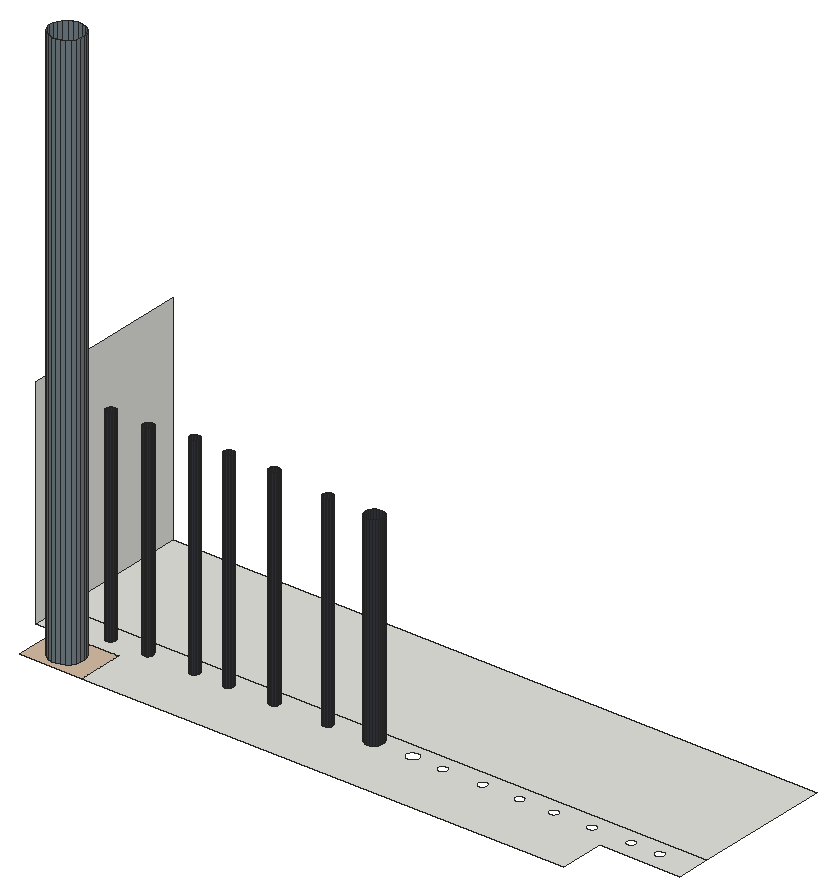
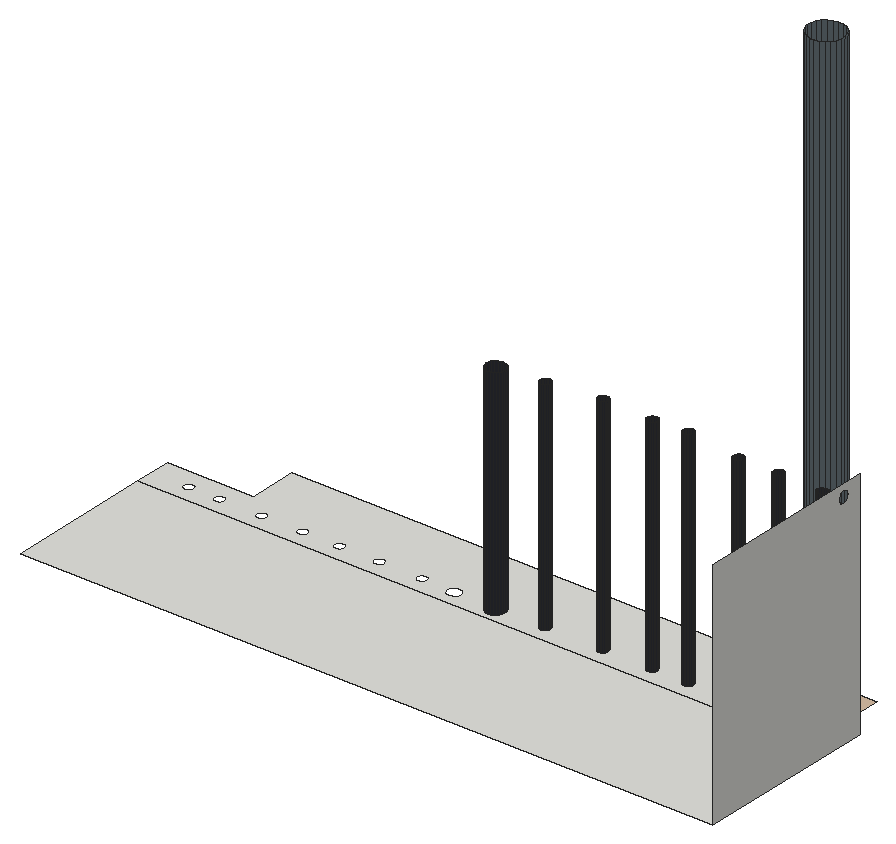
# SketchUp Ruby script. Lengths in inches.
U = 1.inch
M = Sketchup.active_model
def pt(a) = Geom::Point3d.new(a.map { |v| v * U })
def face(e, loops, mat)
  f = e.add_face(loops[0].map { |a| pt(a) })
  loops[1..].each { |l| e.add_face(l.map { |a| pt(a) }).erase! }
  f.material = f.back_material = mat if mat
  f
end
# faces: each face lists its corners as indices into pts; further lists are holes
def faces(e, pts, list, mat = nil) = list.each { |f| face(e, (f[0].is_a?(Array) ? f : [f]).map { |l| l.map { |i| pts[i] } }, mat) }
# xy, xz, yz: faces in a plane at the given z, y or x. An outline is a flat list of corners, or four numbers for a rectangle; further outlines are holes
def ring(l) = l.size == 4 ? [[l[0], l[1]], [l[2], l[1]], [l[2], l[3]], [l[0], l[3]]] : l.each_slice(2).to_a
def flat(e, list, mat, &to3) = list.each { |f| face(e, (f[0].is_a?(Array) ? f : [f]).map { |l| ring(l).map { |u, v| to3.(u, v) } }, mat) }
def xy(e, z, list, mat = nil) = flat(e, list, mat) { |x, y| [x, y, z] }
def xz(e, y, list, mat = nil) = flat(e, list, mat) { |x, z| [x, y, z] }
def yz(e, x, list, mat = nil) = flat(e, list, mat) { |y, z| [x, y, z] }
def lines(e, pts, list) = list.each { |a, b| e.add_line(pt(pts[a]), pt(pts[b])) }
# prism: a flat outline (further loops are holes) pulled along v
def prism(e, loops, v, mat = nil)
  f = face(e, loops, mat); d = Geom::Vector3d.new(v.map { |x| x * U })
  f.pushpull(f.normal.samedirection?(d) ? d.length : -d.length)
end
def box(e, o, s, mat = nil) = prism(e, [[o, [o[0] + s[0], o[1], o[2]], [o[0] + s[0], o[1] + s[1], o[2]], [o[0], o[1] + s[1], o[2]]]], [0, 0, s[2]], mat)
def at(x, y, z, deg = 0) = Geom::Transformation.translation(pt([x, y, z])) * Geom::Transformation.rotation(ORIGIN, Z_AXIS, deg.degrees)
def axes(o, x, y, z) = Geom::Transformation.new([*x, 0, *y, 0, *z, 0, *pt(o).to_a, 1])
def part(name) = M.definitions.add(name)
# library, detail: a bought-in or finely detailed component or shape, given as its bounding box
def library(name, o, s) = part(name).tap { |d| box(d.entities, o, s) }
def detail(e, o, s) = box(e.add_group.entities, o, s)
def put(e, d, t, mat = nil) = e.add_instance(d, t).tap { |i| i.material = mat if mat }
def group(e, t, mat = nil) = e.add_group.tap { |g| g.transformation = t; g.material = mat if mat }.entities
root = M.entities
M.materials.add("[Formica Laminate Dark]").color = [50, 53, 60]
M.materials.add("[Formica Laminate Light]").color = [213, 189, 164]
M.materials.add("[Formica Speckled Grey]").color = [112, 125, 132]
xy(root,160.3,[[[303.97,83.29,372.44,83.29,372.44,89.73,383.79,89.73,383.79,94.63,292.1875,94.63,292.1875,89.73,303.97,89.73],[338.06,91.37,337.73,91.41,337.43,91.54,337.17,91.74,336.97,91.99,336.85,92.3,336.81,92.62,336.85,92.94,336.97,93.24,337.17,93.5,337.43,93.7,337.73,93.83,338.06,93.87,338.38,93.83,338.68,93.7,338.94,93.5,339.14,93.24,339.26,92.94,339.31,92.62,339.26,92.3,339.14,91.99,338.94,91.74,338.68,91.54,338.38,91.41],[343.65,91.54,343.41,91.57,343.18,91.66,342.99,91.8125,342.84,92.01,342.75,92.23,342.71,92.47,342.75,92.72,342.84,92.94,342.99,93.14,343.18,93.29,343.41,93.38,343.65,93.41,343.89,93.38,344.12,93.29,344.31,93.14,344.46,92.94,344.56,92.72,344.59,92.47,344.56,92.23,344.46,92.01,344.31,91.8125,344.12,91.66,343.89,91.57],[331.72,91.61,331.54,91.64,331.375,91.7,331.23,91.8125,331.125,91.96,331.06,92.12,331.03,92.3,331.06,92.48,331.125,92.64,331.23,92.79,331.375,92.89,331.54,92.96,331.72,92.99,331.9,92.96,332.0625,92.89,332.21,92.79,332.32,92.64,332.38,92.48,332.41,92.3,332.38,92.12,332.32,91.96,332.21,91.8125,332.0625,91.7,331.9,91.64],[324.09,91.61,323.92,91.64,323.75,91.7,323.61,91.8125,323.5,91.96,323.43,92.12,323.41,92.3,323.43,92.48,323.5,92.64,323.61,92.79,323.75,92.89,323.92,92.96,324.09,92.99,324.27,92.96,324.4375,92.89,324.58,92.79,324.69,92.64,324.76,92.48,324.78,92.3,324.76,92.12,324.69,91.96,324.58,91.8125,324.4375,91.7,324.27,91.64],[317.59,91.61,317.42,91.64,317.25,91.7,317.11,91.8125,317,91.96,316.93,92.12,316.91,92.3,316.93,92.48,317,92.64,317.11,92.79,317.25,92.89,317.42,92.96,317.59,92.99,317.77,92.96,317.9375,92.89,318.08,92.79,318.19,92.64,318.26,92.48,318.28,92.3,318.26,92.12,318.19,91.96,318.08,91.8125,317.9375,91.7,317.77,91.64],[295.09,91.61,294.92,91.64,294.75,91.7,294.61,91.8125,294.5,91.96,294.43,92.12,294.41,92.3,294.43,92.48,294.5,92.64,294.61,92.79,294.75,92.89,294.92,92.96,295.09,92.99,295.27,92.96,295.4375,92.89,295.58,92.79,295.69,92.64,295.76,92.48,295.78,92.3,295.76,92.12,295.69,91.96,295.58,91.8125,295.4375,91.7,295.27,91.64],[300.84,91.61,300.67,91.64,300.5,91.7,300.36,91.8125,300.25,91.96,300.18,92.12,300.16,92.3,300.18,92.48,300.25,92.64,300.36,92.79,300.5,92.89,300.67,92.96,300.84,92.99,301.02,92.96,301.1875,92.89,301.33,92.79,301.44,92.64,301.51,92.48,301.53,92.3,301.51,92.12,301.44,91.96,301.33,91.8125,301.1875,91.7,301.02,91.64],[306.16,91.61,305.98,91.64,305.8125,91.7,305.67,91.8125,305.5625,91.96,305.49,92.12,305.47,92.3,305.49,92.48,305.5625,92.64,305.67,92.79,305.8125,92.89,305.98,92.96,306.16,92.99,306.34,92.96,306.5,92.89,306.64,92.79,306.75,92.64,306.82,92.48,306.84,92.3,306.82,92.12,306.75,91.96,306.64,91.8125,306.5,91.7,306.34,91.64],[312.78,91.61,312.6,91.64,312.4375,91.7,312.3,91.8125,312.1875,91.96,312.12,92.12,312.09,92.3,312.12,92.48,312.1875,92.64,312.3,92.79,312.4375,92.89,312.6,92.96,312.78,92.99,312.96,92.96,313.125,92.89,313.27,92.79,313.38,92.64,313.45,92.48,313.47,92.3,313.45,92.12,313.38,91.96,313.27,91.8125,313.125,91.7,312.96,91.64],[348.06,91.61,347.88,91.64,347.72,91.7,347.57,91.8125,347.46,91.96,347.4,92.12,347.37,92.3,347.4,92.48,347.46,92.64,347.57,92.79,347.72,92.89,347.88,92.96,348.06,92.99,348.24,92.96,348.4,92.89,348.55,92.79,348.65,92.64,348.72,92.48,348.75,92.3,348.72,92.12,348.65,91.96,348.55,91.8125,348.4,91.7,348.24,91.64],[378.93,91.61,378.76,91.64,378.59,91.7,378.45,91.8125,378.34,91.96,378.27,92.12,378.25,92.3,378.27,92.48,378.34,92.64,378.45,92.79,378.59,92.89,378.76,92.96,378.93,92.99,379.11,92.96,379.28,92.89,379.42,92.79,379.53,92.64,379.6,92.48,379.62,92.3,379.6,92.12,379.53,91.96,379.42,91.8125,379.28,91.7,379.11,91.64],[353.72,91.61,353.54,91.64,353.375,91.7,353.23,91.8125,353.125,91.96,353.06,92.12,353.03,92.3,353.06,92.48,353.125,92.64,353.23,92.79,353.375,92.89,353.54,92.96,353.72,92.99,353.9,92.96,354.0625,92.89,354.21,92.79,354.32,92.64,354.38,92.48,354.41,92.3,354.38,92.12,354.32,91.96,354.21,91.8125,354.0625,91.7,353.9,91.64],[374.84,91.61,374.67,91.64,374.5,91.7,374.36,91.8125,374.25,91.96,374.18,92.12,374.16,92.3,374.18,92.48,374.25,92.64,374.36,92.79,374.5,92.89,374.67,92.96,374.84,92.99,375.02,92.96,375.1875,92.89,375.33,92.79,375.44,92.64,375.51,92.48,375.53,92.3,375.51,92.12,375.44,91.96,375.33,91.8125,375.1875,91.7,375.02,91.64],[358.97,91.61,358.79,91.64,358.625,91.7,358.48,91.8125,358.375,91.96,358.31,92.12,358.28,92.3,358.31,92.48,358.375,92.64,358.48,92.79,358.625,92.89,358.79,92.96,358.97,92.99,359.15,92.96,359.3125,92.89,359.46,92.79,359.57,92.64,359.63,92.48,359.66,92.3,359.63,92.12,359.57,91.96,359.46,91.8125,359.3125,91.7,359.15,91.64],[369.28,91.61,369.1,91.64,368.9375,91.7,368.8,91.8125,368.6875,91.96,368.62,92.12,368.59,92.3,368.62,92.48,368.6875,92.64,368.8,92.79,368.9375,92.89,369.1,92.96,369.28,92.99,369.46,92.96,369.625,92.89,369.77,92.79,369.88,92.64,369.95,92.48,369.97,92.3,369.95,92.12,369.88,91.96,369.77,91.8125,369.625,91.7,369.46,91.64],[363.84,91.61,363.67,91.64,363.5,91.7,363.36,91.8125,363.25,91.96,363.18,92.12,363.16,92.3,363.18,92.48,363.25,92.64,363.36,92.79,363.5,92.89,363.67,92.96,363.84,92.99,364.02,92.96,364.1875,92.89,364.33,92.79,364.44,92.64,364.51,92.48,364.53,92.3,364.51,92.12,364.44,91.96,364.33,91.8125,364.1875,91.7,364.02,91.64]],[298.91,84.16,298.33,84.33,297.8125,84.63,297.39,85.07,297.09,85.59,296.95,86.18,296.95,86.78,297.12,87.36,297.42,87.88,297.86,88.3,298.38,88.6,298.97,88.75,299.57,88.74,300.15,88.58,300.67,88.27,301.09,87.84,301.39,87.3125,301.54,86.73,301.53,86.125,301.37,85.54,301.06,85.02,300.63,84.6,300.1,84.31,299.52,84.16],[338.06,91.37,337.73,91.41,337.43,91.54,337.17,91.74,336.97,91.99,336.85,92.3,336.81,92.62,336.85,92.94,336.97,93.24,337.17,93.5,337.43,93.7,337.73,93.83,338.06,93.87,338.38,93.83,338.68,93.7,338.94,93.5,339.14,93.24,339.26,92.94,339.31,92.62,339.26,92.3,339.14,91.99,338.94,91.74,338.68,91.54,338.38,91.41],[295.09,91.61,294.92,91.64,294.75,91.7,294.61,91.8125,294.5,91.96,294.43,92.12,294.41,92.3,294.43,92.48,294.5,92.64,294.61,92.79,294.75,92.89,294.92,92.96,295.09,92.99,295.27,92.96,295.4375,92.89,295.58,92.79,295.69,92.64,295.76,92.48,295.78,92.3,295.76,92.12,295.69,91.96,295.58,91.8125,295.4375,91.7,295.27,91.64],[306.16,91.61,305.98,91.64,305.8125,91.7,305.67,91.8125,305.5625,91.96,305.49,92.12,305.47,92.3,305.49,92.48,305.5625,92.64,305.67,92.79,305.8125,92.89,305.98,92.96,306.16,92.99,306.34,92.96,306.5,92.89,306.64,92.79,306.75,92.64,306.82,92.48,306.84,92.3,306.82,92.12,306.75,91.96,306.64,91.8125,306.5,91.7,306.34,91.64],
  [312.78,91.61,312.6,91.64,312.4375,91.7,312.3,91.8125,312.1875,91.96,312.12,92.12,312.09,92.3,312.12,92.48,312.1875,92.64,312.3,92.79,312.4375,92.89,312.6,92.96,312.78,92.99,312.96,92.96,313.125,92.89,313.27,92.79,313.38,92.64,313.45,92.48,313.47,92.3,313.45,92.12,313.38,91.96,313.27,91.8125,313.125,91.7,312.96,91.64],[317.59,91.61,317.42,91.64,317.25,91.7,317.11,91.8125,317,91.96,316.93,92.12,316.91,92.3,316.93,92.48,317,92.64,317.11,92.79,317.25,92.89,317.42,92.96,317.59,92.99,317.77,92.96,317.9375,92.89,318.08,92.79,318.19,92.64,318.26,92.48,318.28,92.3,318.26,92.12,318.19,91.96,318.08,91.8125,317.9375,91.7,317.77,91.64],[324.09,91.61,323.92,91.64,323.75,91.7,323.61,91.8125,323.5,91.96,323.43,92.12,323.41,92.3,323.43,92.48,323.5,92.64,323.61,92.79,323.75,92.89,323.92,92.96,324.09,92.99,324.27,92.96,324.4375,92.89,324.58,92.79,324.69,92.64,324.76,92.48,324.78,92.3,324.76,92.12,324.69,91.96,324.58,91.8125,324.4375,91.7,324.27,91.64],[331.72,91.61,331.54,91.64,331.375,91.7,331.23,91.8125,331.125,91.96,331.06,92.12,331.03,92.3,331.06,92.48,331.125,92.64,331.23,92.79,331.375,92.89,331.54,92.96,331.72,92.99,331.9,92.96,332.0625,92.89,332.21,92.79,332.32,92.64,332.38,92.48,332.41,92.3,332.38,92.12,332.32,91.96,332.21,91.8125,332.0625,91.7,331.9,91.64],[292.1875,94.63,383.79,114.1]])
xy(root,160.3,[[[295.13,83.29,303.97,89.73],[298.91,84.16,298.33,84.33,297.8125,84.63,297.39,85.07,297.09,85.59,296.95,86.18,296.95,86.78,297.12,87.36,297.42,87.88,297.86,88.3,298.38,88.6,298.97,88.75,299.57,88.74,300.15,88.58,300.67,88.27,301.09,87.84,301.39,87.3125,301.54,86.73,301.53,86.125,301.37,85.54,301.06,85.02,300.63,84.6,300.1,84.31,299.52,84.16]]],"[Formica Laminate Light]")
xz(root,84.16,[[298.91,160.3,299.52,239.81]],"[Formica Speckled Grey]")
yz(root,292.1875,[[[89.73,160.3,114.1,191.16],[92.39,188.79,92.18,188.82,91.98,188.9,91.82,189.03,91.6875,189.2,91.61,189.39,91.58,189.6,91.61,189.8125,91.6875,190.01,91.82,190.18,91.98,190.31,92.18,190.39,92.39,190.42,92.6,190.39,92.8,190.31,92.96,190.18,93.09,190.01,93.18,189.8125,93.2,189.6,93.18,189.39,93.09,189.2,92.96,189.03,92.8,188.9,92.6,188.82]]])
yz(root,296.95,[[86.18,160.3,86.78,239.81]],"[Formica Speckled Grey]")
p = [[298.33,84.33,160.3],[298.91,84.16,160.3],[298.91,84.16,239.81],[298.33,84.33,239.81],[299.52,84.16,160.3],[300.1,84.31,160.3],
  [300.1,84.31,239.81],[299.52,84.16,239.81],[297.8125,84.63,160.3],[297.8125,84.63,239.81],[300.63,84.6,160.3],[300.63,84.6,239.81],
  [297.39,85.07,160.3],[297.39,85.07,239.81],[301.06,85.02,160.3],[301.06,85.02,239.81],[301.37,85.54,160.3],[301.37,85.54,239.81],
  [297.09,85.59,160.3],[297.09,85.59,239.81],[301.53,86.125,160.3],[301.53,86.125,239.81],[296.95,86.18,160.3],[296.95,86.18,239.81],
  [301.54,86.73,160.3],[301.54,86.73,239.81],[301.39,87.3125,160.3],[301.39,87.3125,239.81],[297.12,87.36,160.3],[296.95,86.78,160.3],
  [296.95,86.78,239.81],[297.12,87.36,239.81],[301.09,87.84,160.3],[301.09,87.84,239.81],[297.42,87.88,160.3],[297.42,87.88,239.81],
  [300.67,88.27,160.3],[300.67,88.27,239.81],[297.86,88.3,160.3],[297.86,88.3,239.81],[298.38,88.6,160.3],[298.38,88.6,239.81],
  [300.15,88.58,160.3],[300.15,88.58,239.81],[298.97,88.75,160.3],[298.97,88.75,239.81],[299.57,88.74,160.3],[299.57,88.74,239.81],
  [337.43,91.54,160.3],[337.73,91.41,160.3],[337.73,91.41,189.05],[337.43,91.54,189.05],[338.06,91.37,160.3],[338.06,91.37,189.05],
  [338.38,91.41,160.3],[338.38,91.41,189.05],[338.68,91.54,160.3],[338.68,91.54,189.05],[337.17,91.74,160.3],[337.17,91.74,189.05],
  [338.94,91.74,160.3],[338.94,91.74,189.05],[294.75,91.7,160.3],[294.92,91.64,160.3],[294.92,91.64,189.24],[294.75,91.7,189.24],
  [295.09,91.61,160.3],[295.09,91.61,189.24],[295.27,91.64,160.3],[295.27,91.64,189.24],[295.4375,91.7,160.3],[295.4375,91.7,189.24],
  [300.5,91.7,160.3],[300.67,91.64,160.3],[300.67,91.64,189.42],[300.5,91.7,189.42],[300.84,91.61,160.3],[300.84,91.61,189.42],
  [301.02,91.64,160.3],[301.02,91.64,189.42],[301.1875,91.7,160.3],[301.1875,91.7,189.42],[305.8125,91.7,160.3],[305.98,91.64,160.3],
  [305.98,91.64,189.36],[305.8125,91.7,189.36],[306.16,91.61,160.3],[306.16,91.61,189.36],[306.34,91.64,160.3],[306.34,91.64,189.36],
  [306.5,91.7,160.3],[306.5,91.7,189.36],[312.4375,91.7,160.3],[312.6,91.64,160.3],[312.6,91.64,190.11],[312.4375,91.7,190.11],
  [312.78,91.61,160.3],[312.78,91.61,190.11],[312.96,91.64,160.3],[312.96,91.64,190.11],[313.125,91.7,160.3],[313.125,91.7,190.11],
  [317.25,91.7,160.3],[317.42,91.64,160.3],[317.42,91.64,189.86],[317.25,91.7,189.86],[317.59,91.61,160.3],[317.59,91.61,189.86],
  [317.77,91.64,160.3],[317.77,91.64,189.86],[317.9375,91.7,160.3],[317.9375,91.7,189.86],[323.75,91.7,160.3],[323.92,91.64,160.3],
  [323.92,91.64,190.01],[323.79,91.6875,190.01],[323.75,91.7,190.01],[324.09,91.61,160.3],[324.09,91.61,190.01],[324.27,91.64,160.3],
  [324.27,91.64,190.01],[324.4375,91.7,160.3],[324.4375,91.7,190.01],[324.4,91.6875,190.01],[331.375,91.7,160.3],[331.54,91.64,160.3],
  [331.54,91.64,189.36],[331.375,91.7,189.36],[331.72,91.61,160.3],[331.72,91.61,189.36],[331.9,91.64,160.3],[331.9,91.64,189.36],
  [332.0625,91.7,160.3],[332.0625,91.7,189.36],[294.61,91.8125,160.3],[294.61,91.8125,189.24],[295.58,91.8125,160.3],[295.58,91.8125,189.24],
  [300.36,91.8125,160.3],[300.36,91.8125,189.42],[301.33,91.8125,160.3],[301.33,91.8125,189.42],[305.67,91.8125,160.3],[305.67,91.8125,189.36],
  [306.64,91.8125,160.3],[306.64,91.8125,189.36],[312.3,91.8125,160.3],[312.3,91.8125,190.11],[313.27,91.8125,160.3],[313.27,91.8125,190.11],
  [317.11,91.8125,160.3],[317.11,91.8125,189.86],[318.08,91.8125,160.3],[318.08,91.8125,189.86],[323.61,91.8125,160.3],[323.61,91.8125,190.01],
  [324.58,91.8125,160.3],[324.58,91.8125,190.01],[331.23,91.8125,160.3],[331.23,91.8125,189.36],[332.21,91.8125,160.3],[332.21,91.8125,189.36],
  [336.97,91.99,160.3],[336.97,91.99,189.05],[339.14,91.99,160.3],[339.14,91.99,189.05],[294.5,91.96,160.3],[294.5,91.96,189.24],
  [295.69,91.96,160.3],[295.69,91.96,189.24],[300.25,91.96,160.3],[300.25,91.96,189.42],[301.44,91.96,160.3],[301.44,91.96,189.42],
  [305.5625,91.96,160.3],[305.5625,91.96,189.36],[306.75,91.96,160.3],[306.75,91.96,189.36],[312.1875,91.96,160.3],[312.1875,91.96,190.11],
  [313.38,91.96,160.3],[313.38,91.96,190.11],[317,91.96,160.3],[317,91.96,189.86],[318.19,91.96,160.3],[318.19,91.96,189.86],
  [323.5,91.96,160.3],[323.5,91.96,190.01],[324.69,91.96,160.3],[324.69,91.96,190.01],[331.125,91.96,160.3],[331.125,91.96,189.36],
  [332.32,91.96,160.3],[332.32,91.96,189.36],[294.43,92.12,160.3],[294.43,92.12,189.24],[295.76,92.12,160.3],[295.76,92.12,189.24],
  [300.18,92.12,160.3],[300.18,92.12,189.42],[301.51,92.12,160.3],[301.51,92.12,189.42],[305.49,92.12,160.3],[305.49,92.12,189.36],
  [306.82,92.12,160.3],[306.82,92.12,189.36],[312.12,92.12,160.3],[312.12,92.12,190.11],[313.45,92.12,160.3],[313.45,92.12,190.11],
  [316.93,92.12,160.3],[316.93,92.12,189.86],[318.26,92.12,160.3],[318.26,92.12,189.86],[323.43,92.12,160.3],[323.43,92.12,190.01],
  [324.76,92.12,160.3],[324.76,92.12,190.01],[331.06,92.12,160.3],[331.06,92.12,189.36],[332.38,92.12,160.3],[332.38,92.12,189.36],
  [336.85,92.3,160.3],[336.85,92.3,189.05],[339.26,92.3,160.3],[339.26,92.3,189.05],[294.41,92.3,160.3],[294.41,92.3,189.24],
  [295.78,92.3,160.3],[295.78,92.3,189.24],[300.16,92.3,160.3],[300.16,92.3,189.42],[301.53,92.3,160.3],[301.53,92.3,189.42],
  [305.47,92.3,160.3],[305.47,92.3,189.36],[306.84,92.3,160.3],[306.84,92.3,189.36],[312.09,92.3,160.3],[312.09,92.3,190.11],
  [313.47,92.3,160.3],[313.47,92.3,190.11],[316.91,92.3,160.3],[316.91,92.3,189.86],[318.28,92.3,160.3],[318.28,92.3,189.86],
  [323.41,92.3,160.3],[323.41,92.3,190.01],[324.78,92.3,160.3],[324.78,92.3,190.01],[331.03,92.3,160.3],[331.03,92.3,189.36],
  [332.41,92.3,160.3],[332.41,92.3,189.36],[294.43,92.48,160.3],[294.43,92.48,189.24],[295.76,92.48,160.3],[295.76,92.48,189.24],
  [300.18,92.48,160.3],[300.18,92.48,189.42],[301.51,92.48,160.3],[301.51,92.48,189.42],[305.49,92.48,160.3],[305.49,92.48,189.36],
  [306.82,92.48,160.3],[306.82,92.48,189.36],[312.12,92.48,160.3],[312.12,92.48,190.11],[313.45,92.48,160.3],[313.45,92.48,190.11],
  [316.93,92.48,160.3],[316.93,92.48,189.86],[318.26,92.48,160.3],[318.26,92.48,189.86],[323.43,92.48,160.3],[323.43,92.48,190.01],
  [324.76,92.48,160.3],[324.76,92.48,190.01],[331.06,92.48,160.3],[331.06,92.48,189.36],[332.38,92.48,160.3],[332.38,92.48,189.36],
  [336.81,92.62,160.3],[336.81,92.62,189.05],[339.31,92.62,160.3],[339.31,92.62,189.05],[294.5,92.64,160.3],[294.5,92.64,189.24],
  [295.69,92.64,160.3],[295.69,92.64,189.24],[300.25,92.64,160.3],[300.25,92.64,189.42],[301.44,92.64,160.3],[301.44,92.64,189.42],
  [305.5625,92.64,160.3],[305.5625,92.64,189.36],[306.75,92.64,160.3],[306.75,92.64,189.36],[312.1875,92.64,160.3],[312.1875,92.64,190.11],
  [313.38,92.64,160.3],[313.38,92.64,190.11],[317,92.64,160.3],[317,92.64,189.86],[318.19,92.64,160.3],[318.19,92.64,189.86],
  [323.5,92.64,160.3],[323.5,92.64,190.01],[324.69,92.64,160.3],[324.69,92.64,190.01],[331.125,92.64,160.3],[331.125,92.64,189.36],
  [332.32,92.64,160.3],[332.32,92.64,189.36],[294.61,92.79,160.3],[294.61,92.79,189.24],[295.58,92.79,160.3],[295.58,92.79,189.24],
  [300.36,92.79,160.3],[300.36,92.79,189.42],[301.33,92.79,160.3],[301.33,92.79,189.42],[305.67,92.79,160.3],[305.67,92.79,189.36],
  [306.64,92.79,160.3],[306.64,92.79,189.36],[312.3,92.79,160.3],[312.3,92.79,190.11],[313.27,92.79,160.3],[313.27,92.79,190.11],
  [317.11,92.79,160.3],[317.11,92.79,189.86],[318.08,92.79,160.3],[318.08,92.79,189.86],[323.61,92.79,160.3],[323.61,92.79,190.01],
  [324.58,92.79,160.3],[324.58,92.79,190.01],[331.23,92.79,160.3],[331.23,92.79,189.36],[332.21,92.79,160.3],[332.21,92.79,189.36],
  [336.85,92.94,160.3],[336.85,92.94,189.05],[339.26,92.94,160.3],[339.26,92.94,189.05],[294.75,92.89,160.3],[294.75,92.89,189.24],
  [295.4375,92.89,160.3],[295.4375,92.89,189.24],[300.5,92.89,160.3],[300.5,92.89,189.42],[301.1875,92.89,160.3],[301.1875,92.89,189.42],
  [305.8125,92.89,160.3],[305.8125,92.89,189.36],[306.5,92.89,160.3],[306.5,92.89,189.36],[312.4375,92.89,160.3],[312.4375,92.89,190.11],
  [313.125,92.89,160.3],[313.125,92.89,190.11],[317.25,92.89,160.3],[317.25,92.89,189.86],[317.9375,92.89,160.3],[317.9375,92.89,189.86],
  [323.75,92.89,160.3],[323.75,92.89,190.01],[324.4375,92.89,160.3],[324.4375,92.89,190.01],[331.375,92.89,160.3],[331.375,92.89,189.36],
  [332.0625,92.89,160.3],[332.0625,92.89,189.36],[294.92,92.96,160.3],[294.92,92.96,189.24],[295.27,92.96,160.3],[295.27,92.96,189.24],
  [300.67,92.96,160.3],[300.67,92.96,189.42],[301.02,92.96,160.3],[301.02,92.96,189.42],[305.98,92.96,160.3],[305.98,92.96,189.36],
  [306.34,92.96,160.3],[306.34,92.96,189.36],[312.6,92.96,160.3],[312.6,92.96,190.11],[312.96,92.96,160.3],[312.96,92.96,190.11],
  [317.42,92.96,160.3],[317.42,92.96,189.86],[317.77,92.96,160.3],[317.77,92.96,189.86],[323.92,92.96,160.3],[323.92,92.96,190.01],
  [324.27,92.96,160.3],[324.27,92.96,190.01],[331.54,92.96,160.3],[331.54,92.96,189.36],[331.9,92.96,160.3],[331.9,92.96,189.36],
  [336.97,93.24,160.3],[336.97,93.24,189.05],[339.14,93.24,160.3],[339.14,93.24,189.05],[295.09,92.99,160.3],[295.09,92.99,189.24],
  [300.84,92.99,160.3],[300.84,92.99,189.42],[306.16,92.99,160.3],[306.16,92.99,189.36],[312.78,92.99,160.3],[312.78,92.99,190.11],
  [317.59,92.99,160.3],[317.59,92.99,189.86],[324.09,92.99,160.3],[324.09,92.99,190.01],[331.72,92.99,160.3],[331.72,92.99,189.36],
  [337.17,93.5,160.3],[337.17,93.5,189.05],[338.94,93.5,160.3],[338.94,93.5,189.05],[337.43,93.7,160.3],[337.43,93.7,189.05],
  [338.68,93.7,160.3],[338.68,93.7,189.05],[337.73,93.83,160.3],[337.73,93.83,189.05],[338.38,93.83,160.3],[338.38,93.83,189.05],
  [338.06,93.87,160.3],[338.06,93.87,189.05]]
faces(root,p,[[0,1,2,3],[4,5,6,7],[8,0,3,9],[5,10,11,6],[12,8,9,13],[10,14,15,11],[14,16,17,15],[18,12,13,19],
  [16,20,21,17],[22,18,19,23],[20,24,25,21],[24,26,27,25],[28,29,30,31],[26,32,33,27],[34,28,31,35],[32,36,37,33],
  [38,34,35,39],[40,38,39,41],[36,42,43,37],[44,40,41,45],[42,46,47,43],[46,44,45,47]],"[Formica Speckled Grey]")
faces(root,p,[[48,49,50,51],[49,52,53,50],[52,54,55,53],[54,56,57,55],[58,48,51,59],[56,60,61,57],[62,63,64,65],[63,66,67,64],
  [66,68,69,67],[68,70,71,69],[72,73,74,75],[73,76,77,74],[76,78,79,77],[78,80,81,79],[82,83,84,85],[83,86,87,84],
  [86,88,89,87],[88,90,91,89],[92,93,94,95],[93,96,97,94],[96,98,99,97],[98,100,101,99],[102,103,104,105],[103,106,107,104],
  [106,108,109,107],[108,110,111,109],[112,113,114,115,116],[113,117,118,114],[117,119,120,118],[119,121,122,123,120],[124,125,126,127],[125,128,129,126],
  [128,130,131,129],[130,132,133,131],[134,62,65,135],[70,136,137,71],[138,72,75,139],[80,140,141,81],[142,82,85,143],[90,144,145,91],
  [146,92,95,147],[100,148,149,101],[150,102,105,151],[110,152,153,111],[154,112,116,155],[121,156,157,122],[158,124,127,159],[132,160,161,133],
  [162,58,59,163],[60,164,165,61],[166,134,135,167],[136,168,169,137],[170,138,139,171],[140,172,173,141],[174,142,143,175],[144,176,177,145],
  [178,146,147,179],[148,180,181,149],[182,150,151,183],[152,184,185,153],[186,154,155,187],[156,188,189,157],[190,158,159,191],[160,192,193,161],
  [194,166,167,195],[168,196,197,169],[198,170,171,199],[172,200,201,173],[202,174,175,203],[176,204,205,177],[206,178,179,207],[180,208,209,181],
  [210,182,183,211],[184,212,213,185],[214,186,187,215],[188,216,217,189],[218,190,191,219],[192,220,221,193],[222,162,163,223],[164,224,225,165],
  [226,194,195,227],[196,228,229,197],[230,198,199,231],[200,232,233,201],[234,202,203,235],[204,236,237,205],[238,206,207,239],[208,240,241,209],
  [242,210,211,243],[212,244,245,213],[246,214,215,247],[216,248,249,217],[250,218,219,251],[220,252,253,221],[254,226,227,255],[228,256,257,229],
  [258,230,231,259],[232,260,261,233],[262,234,235,263],[236,264,265,237],[266,238,239,267],[240,268,269,241],[270,242,243,271],[244,272,273,245],
  [274,246,247,275],[248,276,277,249],[278,250,251,279],[252,280,281,253],[282,222,223,283],[224,284,285,225],[286,254,255,287],[256,288,289,257],
  [290,258,259,291],[260,292,293,261],[294,262,263,295],[264,296,297,265],[298,266,267,299],[268,300,301,269],[302,270,271,303],[272,304,305,273],
  [306,274,275,307],[276,308,309,277],[310,278,279,311],[280,312,313,281],[314,286,287,315],[288,316,317,289],[318,290,291,319],[292,320,321,293],
  [322,294,295,323],[296,324,325,297],[326,298,299,327],[300,328,329,301],[330,302,303,331],[304,332,333,305],[334,306,307,335],[308,336,337,309],
  [338,310,311,339],[312,340,341,313],[342,282,283,343],[284,344,345,285],[346,314,315,347],[316,348,349,317],[350,318,319,351],[320,352,353,321],
  [354,322,323,355],[324,356,357,325],[358,326,327,359],[328,360,361,329],[362,330,331,363],[332,364,365,333],[366,334,335,367],[336,368,369,337],
  [370,338,339,371],[340,372,373,341],[374,346,347,375],[348,376,377,349],[378,350,351,379],[352,380,381,353],[382,354,355,383],[356,384,385,357],
  [386,358,359,387],[360,388,389,361],[390,362,363,391],[364,392,393,365],[394,366,367,395],[368,396,397,369],[398,370,371,399],[372,400,401,373],
  [402,342,343,403],[344,404,405,345],[406,374,375,407],[376,406,407,377],[408,378,379,409],[380,408,409,381],[410,382,383,411],[384,410,411,385],
  [412,386,387,413],[388,412,413,389],[414,390,391,415],[392,414,415,393],[416,394,395,417],[396,416,417,397],[418,398,399,419],[400,418,419,401],
  [420,402,403,421],[404,422,423,405],[424,420,421,425],[422,426,427,423],[428,424,425,429],[426,430,431,427],[432,428,429,433],[430,432,433,431]],"[Formica Laminate Dark]")
